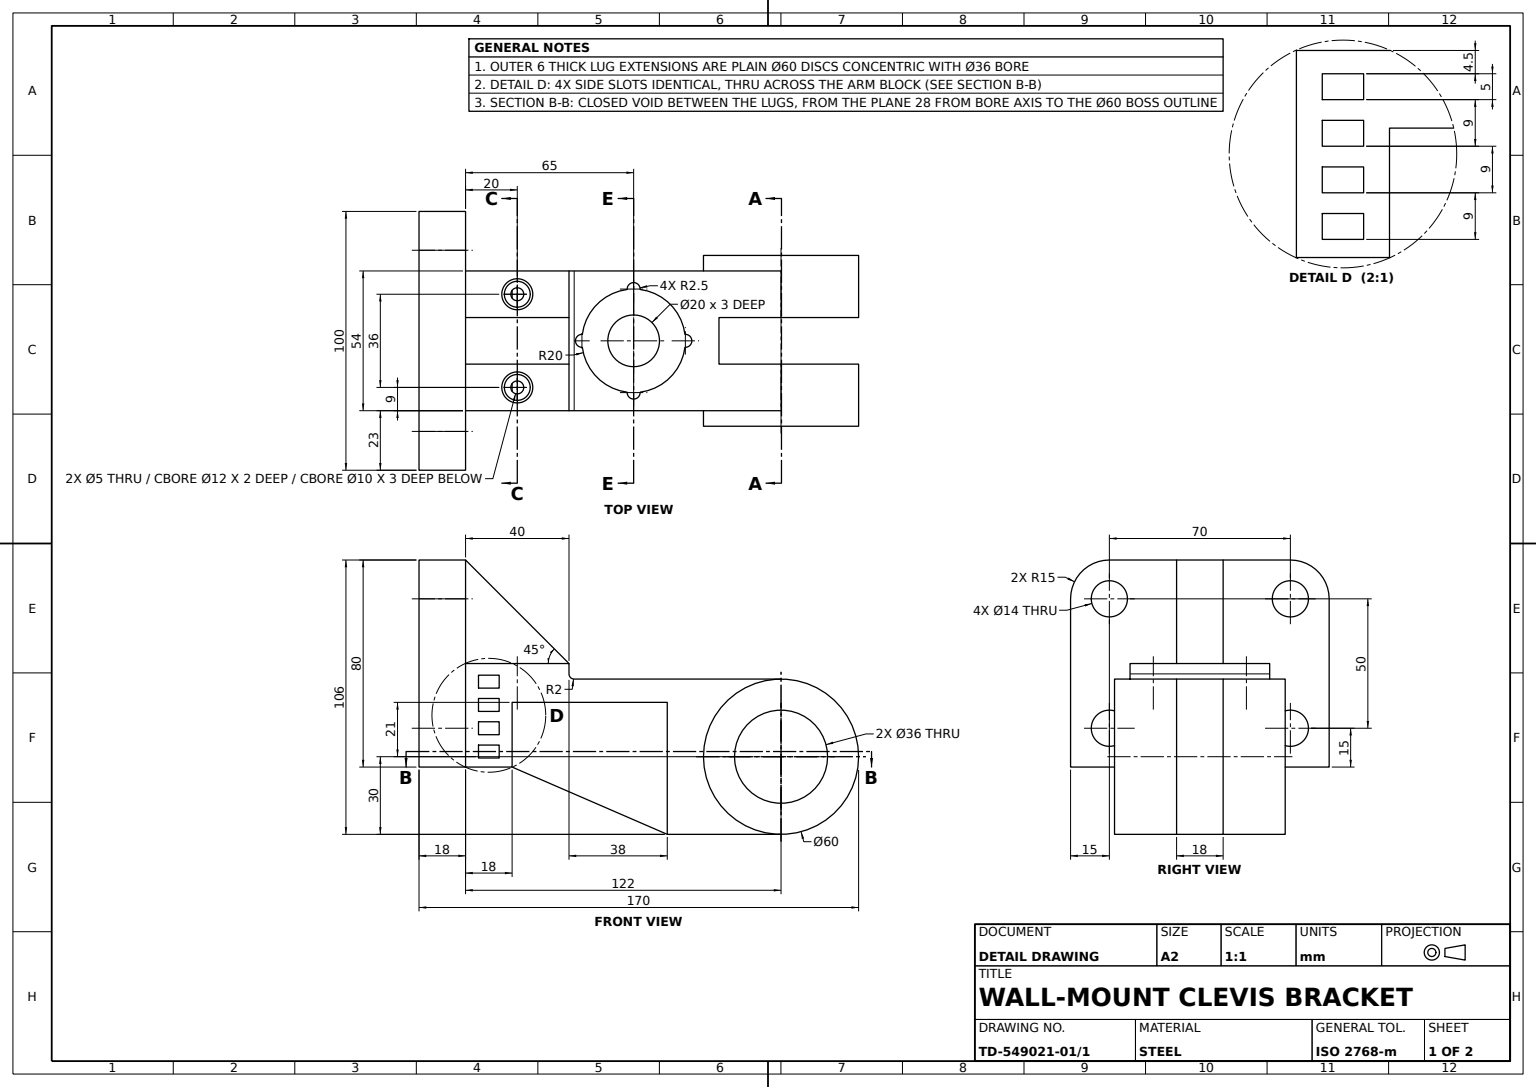
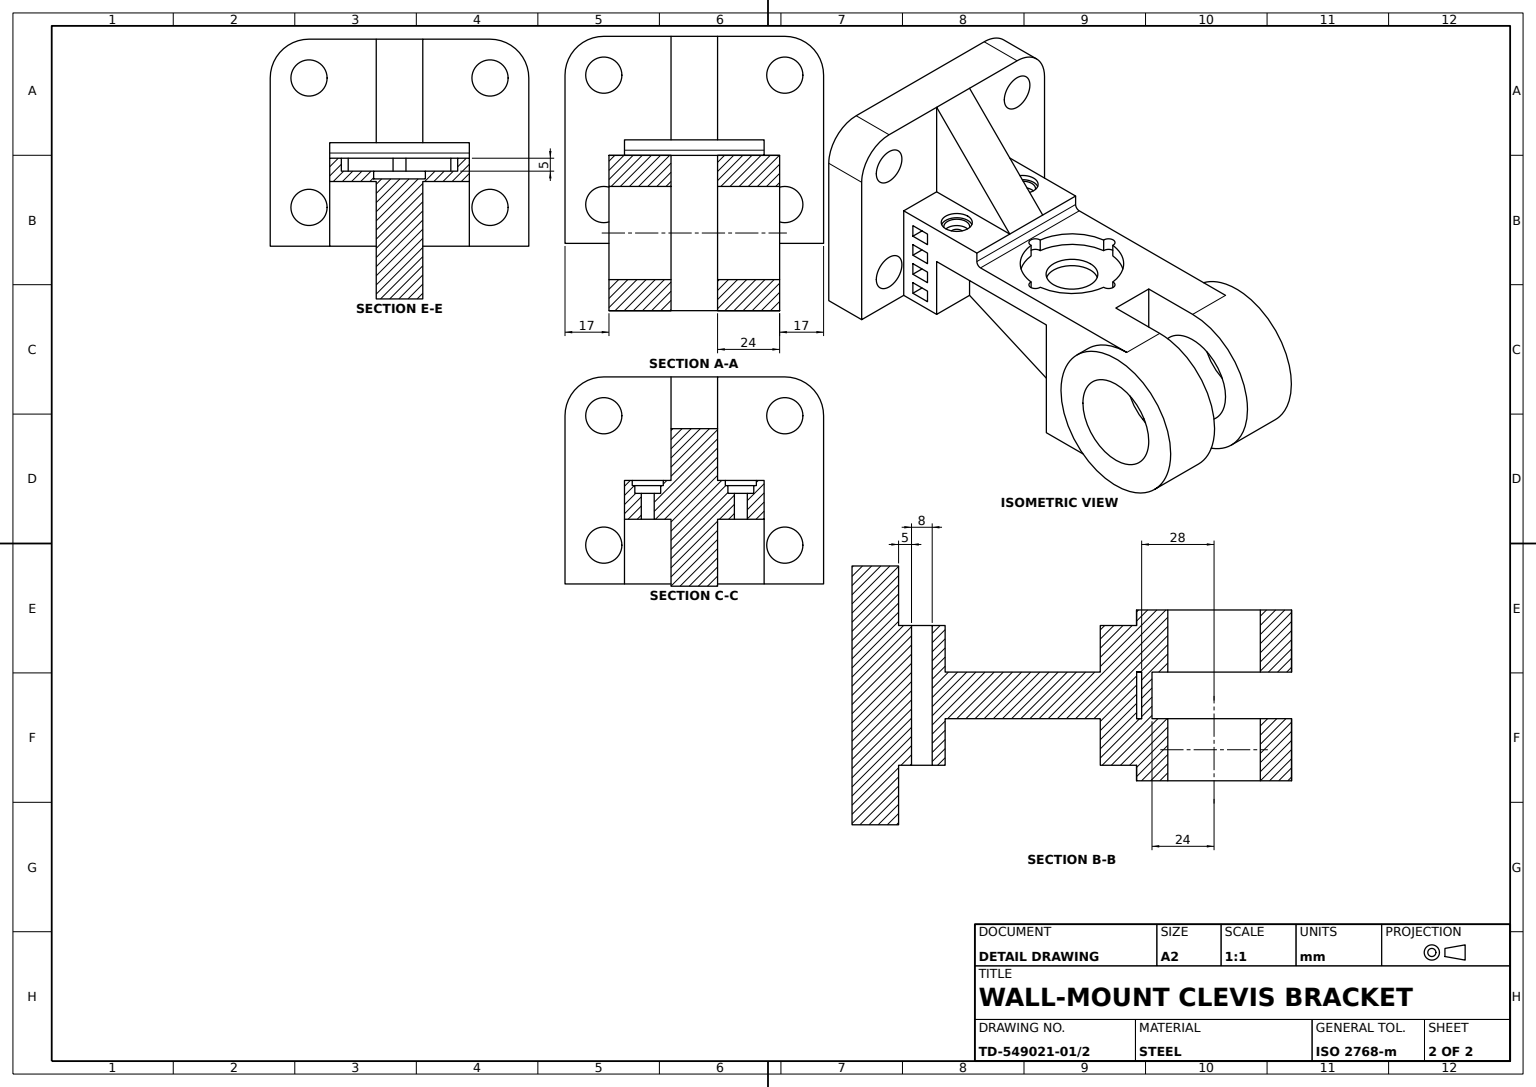
solid
v1 (38,-2,-12)
v2 (38,-2,-24)
e1 v1 v2 CIRCLE(AX(P(38,-2,-18),D(0,1,0),D(0,0,1)),6)
e2 v2 v1 CIRCLE(AX(P(38,-2,-18),D(0,1,0),D(0,0,1)),6)
v3 (38,-2,-23)
v4 (38,-2,-13)
e3 v3 v4 CIRCLE(AX(P(38,-2,-18),D(0,-1,0),D(0,0,1)),5)
e4 v4 v3 CIRCLE(AX(P(38,-2,-18),D(0,-1,0),D(0,0,1)),5)
face PLANE(AX(P(38,-2,-18),D(0,1,0),D(0,0,1))) [e1 e2] [e3 e4]
v5 (38,-5,-13)
v6 (38,-5,-23)
e5 v5 v6 CIRCLE(AX(P(38,-5,-18),D(0,1,0),D(0,0,1)),5)
e6 v5 v4 LINE
e7 v6 v3 LINE
face CYL(AX(P(38,-5,-18),D(0,1,0),D(0,0,1)),5) rev [-e5 e6 -e3 -e7]
v7 (0,25,-28)
v8 (18,25,-28)
e8 v7 v8 LINE
v9 (18,25,-42)
e9 v8 v9 CIRCLE(AX(P(18,25,-35),D(1,0,0),D(0,0,-1)),7)
v10 (0,25,-42)
e10 v10 v9 LINE
e11 v7 v10 CIRCLE(AX(P(0,25,-35),D(1,0,0),D(0,0,-1)),7)
face CYL(AX(P(0,25,-35),D(1,0,0),D(0,0,-1)),7) rev [e8 e9 -e10 -e11]
v11 (85.495112,-11,-19.84375)
v12 (85.495112,-6,-19.84375)
e12 v11 v12 LINE
v13 (80.504888,-6,-19.84375)
e13 v12 v13 CIRCLE(AX(P(83,-6,-20),D(0,1,0),D(0,0,1)),2.5)
v14 (80.504888,-11,-19.84375)
e14 v14 v13 LINE
e15 v11 v14 CIRCLE(AX(P(83,-11,-20),D(0,1,0),D(0,0,1)),2.5)
face CYL(AX(P(83,-11,-20),D(0,1,0),D(0,0,1)),2.5) rev [e12 e13 -e14 -e15]
v15 (96,-15,9)
v16 (96,-15,27)
e16 v15 v16 LINE
v17 (96,-66,9)
e17 v17 v15 LINE
v18 (96,-66,27)
e18 v17 v18 LINE
e19 v16 v18 LINE
face PLANE(AX(P(96,0,-27),D(-1,0,0),D(0,0,1))) [-e16 -e17 e18 -e19]
v19 (38,-15,-20.5)
v20 (38,-5,-20.5)
e20 v19 v20 LINE
v21 (38,-15,-15.5)
e21 v21 v19 CIRCLE(AX(P(38,-15,-18),D(0,1,0),D(0,0,1)),2.5)
v22 (38,-5,-15.5)
e22 v21 v22 LINE
e23 v20 v22 CIRCLE(AX(P(38,-5,-18),D(0,-1,0),D(0,0,1)),2.5)
face CYL(AX(P(38,-15,-18),D(0,1,0),D(0,0,1)),2.5) rev [-e20 -e21 e22 -e23]
v23 (85.495112,-6,19.84375)
v24 (102.84375,-6,2.495112)
e24 v23 v24 CIRCLE(AX(P(83,-6,0),D(0,1,0),D(0,0,1)),20)
v25 (102.84375,-11,2.495112)
e25 v25 v24 LINE
v26 (85.495112,-11,19.84375)
e26 v26 v25 CIRCLE(AX(P(83,-11,0),D(0,1,0),D(0,0,1)),20)
e27 v26 v23 LINE
face CYL(AX(P(83,-11,0),D(0,1,0),D(0,0,1)),20) rev [e24 -e25 -e26 e27]
v27 (38,0,-12)
e28 v1 v27 LINE
v28 (38,0,-24)
e29 v27 v28 CIRCLE(AX(P(38,0,-18),D(0,1,0),D(0,0,1)),6)
e30 v2 v28 LINE
face CYL(AX(P(38,-2,-18),D(0,1,0),D(0,0,1)),6) rev [-e1 e28 e29 -e30]
v29 (38,-2,12)
v30 (38,0,12)
e31 v29 v30 LINE
v31 (38,0,24)
e32 v30 v31 CIRCLE(AX(P(38,0,18),D(0,1,0),D(0,0,1)),6)
v32 (38,-2,24)
e33 v32 v31 LINE
e34 v29 v32 CIRCLE(AX(P(38,-2,18),D(0,1,0),D(0,0,1)),6)
face CYL(AX(P(38,-2,18),D(0,1,0),D(0,0,1)),6) rev [e31 e32 -e33 -e34]
v33 (58,0,9)
v34 (58,0,-9)
e35 v33 v34 LINE
v35 (58,0,27)
e36 v35 v33 LINE
v36 (58,-4,27)
e37 v36 v35 LINE
v37 (58,-4,-27)
e38 v36 v37 LINE
v38 (58,0,-27)
e39 v37 v38 LINE
e40 v34 v38 LINE
face PLANE(AX(P(58,-15,-27),D(1,0,0),D(0,0,-1))) [-e35 -e36 -e37 e38 e39 -e40]
v39 (110,-36,27)
v40 (110,-36,33)
e41 v39 v40 LINE
v41 (140,-66,27)
e42 v39 v41 CIRCLE(AX(P(140,-36,27),D(0,0,1),D(1,0,0)),30)
v42 (140,-66,9)
e43 v42 v41 LINE
v43 (170,-36,9)
e44 v42 v43 CIRCLE(AX(P(140,-36,9),D(0,0,1),D(1,0,0)),30)
v44 (170,-36,33)
e45 v43 v44 LINE
e46 v40 v44 CIRCLE(AX(P(140,-36,33),D(0,0,1),D(1,0,0)),30)
face CYL(AX(P(140,-36,9),D(0,0,1),D(1,0,0)),30) [-e41 e42 -e43 e44 e45 -e46]
v45 (60,-6,27)
e47 v45 v36 CIRCLE(AX(P(60,-4,27),D(0,0,-1),D(-1,0,0)),2)
v46 (60,-6,-27)
e48 v46 v45 LINE
e49 v37 v46 CIRCLE(AX(P(60,-4,-27),D(0,0,1),D(-1,0,0)),2)
face CYL(AX(P(60,-4,-27),D(0,0,-1),D(-1,0,0)),2) rev [-e38 -e47 -e48 -e49]
v47 (0,-25,28)
v48 (18,-25,28)
e50 v47 v48 LINE
v49 (0,-25,42)
e51 v49 v47 CIRCLE(AX(P(0,-25,35),D(1,0,0),D(0,0,-1)),7)
v50 (18,-25,42)
e52 v49 v50 LINE
e53 v50 v48 CIRCLE(AX(P(18,-25,35),D(1,0,0),D(0,0,-1)),7)
face CYL(AX(P(0,-25,35),D(1,0,0),D(0,0,-1)),7) rev [-e50 -e51 e52 e53]
v51 (18,-25,-42)
v52 (18,-25,-28)
e54 v51 v52 CIRCLE(AX(P(18,-25,-35),D(1,0,0),D(0,0,-1)),7)
v53 (0,-25,-28)
e55 v53 v52 LINE
v54 (0,-25,-42)
e56 v54 v53 CIRCLE(AX(P(0,-25,-35),D(1,0,0),D(0,0,-1)),7)
e57 v54 v51 LINE
face CYL(AX(P(0,-25,-35),D(1,0,0),D(0,0,-1)),7) rev [e54 -e55 -e56 e57]
e58 v10 v7 CIRCLE(AX(P(0,25,-35),D(1,0,0),D(0,0,-1)),7)
e59 v9 v8 CIRCLE(AX(P(18,25,-35),D(1,0,0),D(0,0,-1)),7)
face CYL(AX(P(0,25,-35),D(1,0,0),D(0,0,-1)),7) rev [-e58 e10 e59 -e8]
e60 v52 v51 CIRCLE(AX(P(18,-25,-35),D(1,0,0),D(0,0,-1)),7)
v55 (18,0,-27)
v56 (18,-40,-27)
e61 v55 v56 LINE
v57 (18,-40,-50)
e62 v56 v57 LINE
v58 (18,25,-50)
e63 v57 v58 LINE
v59 (18,40,-35)
e64 v58 v59 CIRCLE(AX(P(18,25,-35),D(1,0,0),D(0,0,-1)),15)
v60 (18,40,-9)
e65 v59 v60 LINE
v61 (18,0,-9)
e66 v60 v61 LINE
e67 v55 v61 LINE
face PLANE(AX(P(18,25,35),D(1,0,0),D(0,0,-1))) [-e59 -e9] [-e60 -e54] [e61 e62 e63 e64 e65 e66 -e67]
e68 v53 v54 CIRCLE(AX(P(0,-25,-35),D(1,0,0),D(0,0,-1)),7)
v62 (0,-40,-50)
v63 (0,25,-50)
e69 v62 v63 LINE
v64 (0,-40,50)
e70 v64 v62 LINE
v65 (0,25,50)
e71 v65 v64 LINE
v66 (0,40,35)
e72 v66 v65 CIRCLE(AX(P(0,25,35),D(1,0,0),D(0,0,-1)),15)
v67 (0,40,-35)
e73 v67 v66 LINE
e74 v63 v67 CIRCLE(AX(P(0,25,-35),D(1,0,0),D(0,0,-1)),15)
v68 (0,25,42)
v69 (0,25,28)
e75 v68 v69 CIRCLE(AX(P(0,25,35),D(1,0,0),D(0,0,-1)),7)
e76 v69 v68 CIRCLE(AX(P(0,25,35),D(1,0,0),D(0,0,-1)),7)
e77 v47 v49 CIRCLE(AX(P(0,-25,35),D(1,0,0),D(0,0,-1)),7)
face PLANE(AX(P(0,25,35),D(1,0,0),D(0,0,-1))) rev [e56 e68] [-e69 -e70 -e71 -e72 -e73 -e74] [e11 e58] [e75 e76] [e77 e51]
v70 (18,25,50)
e78 v70 v65 LINE
v71 (18,40,35)
e79 v71 v70 CIRCLE(AX(P(18,25,35),D(1,0,0),D(0,0,-1)),15)
e80 v71 v66 LINE
face CYL(AX(P(18,25,35),D(-1,0,0),D(0,0,1)),15) [-e78 -e79 e80 e72]
v72 (116,-6,9)
v73 (140,-6,9)
e81 v72 v73 LINE
e82 v43 v73 CIRCLE(AX(P(140,-36,9),D(0,0,1),D(1,0,0)),30)
v74 (116,-66,9)
e83 v74 v42 LINE
e84 v74 v72 LINE
v75 (122,-36,9)
v76 (158,-36,9)
e85 v75 v76 CIRCLE(AX(P(140,-36,9),D(0,0,1),D(1,0,0)),18)
e86 v76 v75 CIRCLE(AX(P(140,-36,9),D(0,0,1),D(1,0,0)),18)
face PLANE(AX(P(0,0,9),D(0,0,1),D(1,0,0))) rev [e81 -e82 -e44 -e83 e84] [e85 e86]
v77 (18,0,9)
e87 v33 v77 LINE
v78 (18,0,27)
e88 v77 v78 LINE
e89 v78 v35 LINE
e90 v31 v30 CIRCLE(AX(P(38,0,18),D(0,1,0),D(0,0,1)),6)
face PLANE(AX(P(0,0,0),D(0,-1,0),D(0,0,-1))) rev [e36 e87 e88 e89] [-e32 -e90]
e91 v34 v61 LINE
e92 v55 v38 LINE
e93 v28 v27 CIRCLE(AX(P(38,0,-18),D(0,1,0),D(0,0,1)),6)
face PLANE(AX(P(0,0,0),D(0,-1,0),D(0,0,-1))) rev [-e91 e40 -e92 e67] [-e29 -e93]
v79 (31,-27.5,-27)
v80 (31,-27.5,27)
e94 v79 v80 LINE
v81 (23,-27.5,-27)
e95 v79 v81 LINE
v82 (23,-27.5,27)
e96 v81 v82 LINE
e97 v82 v80 LINE
face PLANE(AX(P(23,-27.5,-50),D(0,-1,0),D(0,0,-1))) rev [-e94 e95 e96 e97]
v83 (122,-36,33)
e98 v75 v83 LINE
v84 (158,-36,33)
e99 v76 v84 LINE
e100 v84 v83 CIRCLE(AX(P(140,-36,33),D(0,0,1),D(1,0,0)),18)
face CYL(AX(P(140,-36,9),D(0,0,1),D(1,0,0)),18) rev [-e98 -e86 e99 e100]
v85 (140,-66,-27)
v86 (140,-66,-9)
e101 v85 v86 LINE
v87 (110,-36,-27)
e102 v85 v87 CIRCLE(AX(P(140,-36,-27),D(0,0,-1),D(-1,0,0)),30)
v88 (110,-36,-33)
e103 v87 v88 LINE
v89 (170,-36,-33)
e104 v89 v88 CIRCLE(AX(P(140,-36,-33),D(0,0,-1),D(-1,0,0)),30)
v90 (170,-36,-9)
e105 v90 v89 LINE
e106 v90 v86 CIRCLE(AX(P(140,-36,-9),D(0,0,-1),D(-1,0,0)),30)
face CYL(AX(P(140,-36,-9),D(0,0,-1),D(-1,0,0)),30) [-e101 e102 e103 -e104 -e105 e106]
v91 (36,-40,-9)
v92 (36,-40,-27)
e107 v91 v92 LINE
v93 (36,-40,9)
e108 v91 v93 LINE
v94 (36,-40,27)
e109 v94 v93 LINE
v95 (18,-40,27)
e110 v95 v94 LINE
v96 (18,-40,50)
e111 v96 v95 LINE
e112 v96 v64 LINE
e113 v57 v62 LINE
e114 v56 v92 LINE
face PLANE(AX(P(18,-40,50),D(0,1,0),D(0,0,1))) rev [-e107 e108 -e109 -e110 -e111 e112 e70 -e113 -e62 e114]
v97 (23,-36.5,-27)
v98 (23,-31.5,-27)
e115 v97 v98 LINE
v99 (23,-31.5,27)
e116 v98 v99 LINE
v100 (23,-36.5,27)
e117 v99 v100 LINE
e118 v97 v100 LINE
face PLANE(AX(P(23,-31.5,-50),D(-1,0,0),D(0,0,1))) rev [e115 e116 e117 -e118]
v101 (96,-66,-27)
e119 v101 v85 LINE
v102 (116,-66,-9)
e120 v86 v102 LINE
e121 v102 v74 LINE
e122 v18 v41 LINE
v103 (96,-66,-9)
e123 v103 v17 LINE
e124 v101 v103 LINE
face PLANE(AX(P(0,-66,-27),D(0,-1,0),D(0,0,-1))) [e119 e101 e120 e121 e83 e43 -e122 -e18 -e123 -e124]
v104 (63.15625,-6,2.495112)
v105 (80.504888,-6,19.84375)
e125 v104 v105 CIRCLE(AX(P(83,-6,0),D(0,1,0),D(0,0,1)),20)
v106 (80.504888,-11,19.84375)
e126 v106 v105 LINE
v107 (63.15625,-11,2.495112)
e127 v107 v106 CIRCLE(AX(P(83,-11,0),D(0,1,0),D(0,0,1)),20)
e128 v107 v104 LINE
face CYL(AX(P(83,-11,0),D(0,1,0),D(0,0,1)),20) rev [e125 -e126 -e127 e128]
face CYL(AX(P(38,-2,-18),D(0,1,0),D(0,0,1)),6) rev [e30 e93 -e28 -e2]
v108 (36,-15,16.5)
v109 (36,-15,9)
e129 v108 v109 LINE
e130 v109 v15 LINE
v110 (36,-15,27)
e131 v110 v16 LINE
v111 (36,-15,19.5)
e132 v110 v111 LINE
v112 (38,-15,20.5)
e133 v111 v112 CIRCLE(AX(P(38,-15,18),D(0,1,0),D(0,0,1)),2.5)
v113 (38,-15,15.5)
e134 v112 v113 CIRCLE(AX(P(38,-15,18),D(0,1,0),D(0,0,1)),2.5)
e135 v113 v108 CIRCLE(AX(P(38,-15,18),D(0,1,0),D(0,0,1)),2.5)
face PLANE(AX(P(0,-15,0),D(0,1,0),D(0,0,1))) rev [e129 e130 e16 -e131 e132 e133 e134 e135]
e136 v93 v109 LINE
e137 v93 v17 LINE
face PLANE(AX(P(85,-13,9),D(0,0,1),D(1,0,0))) [-e130 -e136 e137 e17]
v114 (31,-4.5,27)
v115 (23,-4.5,27)
e138 v114 v115 LINE
v116 (31,-9.5,27)
e139 v116 v114 LINE
v117 (23,-9.5,27)
e140 v117 v116 LINE
e141 v115 v117 LINE
v118 (140,-6,27)
e142 v118 v39 CIRCLE(AX(P(140,-36,27),D(0,0,1),D(1,0,0)),30)
e143 v118 v45 LINE
e144 v78 v95 LINE
e145 v110 v94 LINE
v119 (23,-13.5,27)
v120 (23,-18.5,27)
e146 v119 v120 LINE
v121 (31,-13.5,27)
e147 v121 v119 LINE
v122 (31,-18.5,27)
e148 v122 v121 LINE
e149 v120 v122 LINE
v123 (23,-22.5,27)
e150 v123 v82 LINE
v124 (31,-22.5,27)
e151 v124 v123 LINE
e152 v80 v124 LINE
v125 (31,-31.5,27)
e153 v125 v99 LINE
v126 (31,-36.5,27)
e154 v126 v125 LINE
e155 v100 v126 LINE
face PLANE(AX(P(0,0,27),D(0,0,-1),D(-1,0,0))) rev [-e138 -e139 -e140 -e141] [e19 e122 -e42 -e142 e143 e47 e37 -e89 e144 e110 -e145 e131] [-e146 -e147 -e148 -e149] [-e150 -e151 -e152 -e97] [-e117 -e153 -e154 -e155]
e156 v59 v67 LINE
e157 v58 v63 LINE
face CYL(AX(P(18,25,-35),D(-1,0,0),D(0,0,1)),15) [e74 -e156 -e64 e157]
v127 (96,-15,-9)
e158 v103 v127 LINE
v128 (96,-15,-27)
e159 v128 v127 LINE
e160 v128 v101 LINE
face PLANE(AX(P(96,0,-27),D(-1,0,0),D(0,0,1))) [e158 -e159 e160 e124]
v129 (18,40,9)
e161 v129 v71 LINE
e162 v60 v129 LINE
face PLANE(AX(P(18,40,35),D(0,-1,0),D(0,0,-1))) rev [-e161 -e162 -e65 e156 e73 -e80]
v130 (158,-36,-33)
v131 (122,-36,-33)
e163 v130 v131 CIRCLE(AX(P(140,-36,-33),D(0,0,-1),D(-1,0,0)),18)
e164 v131 v130 CIRCLE(AX(P(140,-36,-33),D(0,0,-1),D(-1,0,0)),18)
e165 v88 v89 CIRCLE(AX(P(140,-36,-33),D(0,0,-1),D(-1,0,0)),30)
face PLANE(AX(P(140,-36,-33),D(0,0,-1),D(-1,0,0))) [-e163 -e164] [e104 e165]
v132 (23,-13.5,-27)
e166 v132 v119 LINE
v133 (23,-18.5,-27)
e167 v133 v120 LINE
e168 v133 v132 LINE
face PLANE(AX(P(23,-13.5,-50),D(-1,0,0),D(0,0,1))) rev [e166 e146 -e167 e168]
v134 (103,-6,-2.5)
v135 (102.84375,-6,-2.495112)
e169 v134 v135 CIRCLE(AX(P(103,-6,0),D(0,1,0),D(0,0,1)),2.5)
v136 (102.84375,-11,-2.495112)
e170 v136 v135 LINE
v137 (103,-11,-2.5)
e171 v137 v136 CIRCLE(AX(P(103,-11,0),D(0,1,0),D(0,0,1)),2.5)
e172 v137 v134 LINE
face CYL(AX(P(103,-11,0),D(0,1,0),D(0,0,1)),2.5) rev [e169 -e170 -e171 e172]
v138 (36,-15,-19.5)
e173 v19 v138 CIRCLE(AX(P(38,-15,-18),D(0,1,0),D(0,0,1)),2.5)
v139 (36,-15,-27)
e174 v138 v139 LINE
e175 v128 v139 LINE
v140 (36,-15,-9)
e176 v140 v127 LINE
v141 (36,-15,-16.5)
e177 v140 v141 LINE
e178 v141 v21 CIRCLE(AX(P(38,-15,-18),D(0,1,0),D(0,0,1)),2.5)
face PLANE(AX(P(0,-15,0),D(0,1,0),D(0,0,1))) rev [e21 e173 e174 -e175 e159 -e176 e177 e178]
v142 (83,-6,22.5)
e179 v105 v142 CIRCLE(AX(P(83,-6,20),D(0,1,0),D(0,0,1)),2.5)
v143 (83,-11,22.5)
e180 v143 v142 LINE
e181 v106 v143 CIRCLE(AX(P(83,-11,20),D(0,1,0),D(0,0,1)),2.5)
face CYL(AX(P(83,-11,20),D(0,1,0),D(0,0,1)),2.5) rev [e179 -e180 -e181 e126]
e182 v60 v34 LINE
face PLANE(AX(P(29,0,-9),D(0,0,1),D(1,0,0))) rev [e182 e91 -e66]
e183 v135 v12 CIRCLE(AX(P(83,-6,0),D(0,1,0),D(0,0,1)),20)
e184 v136 v11 CIRCLE(AX(P(83,-11,0),D(0,1,0),D(0,0,1)),20)
face CYL(AX(P(83,-11,0),D(0,1,0),D(0,0,1)),20) rev [e183 -e12 -e184 e170]
v144 (63.15625,-6,-2.495112)
e185 v13 v144 CIRCLE(AX(P(83,-6,0),D(0,1,0),D(0,0,1)),20)
v145 (63.15625,-11,-2.495112)
e186 v145 v144 LINE
e187 v14 v145 CIRCLE(AX(P(83,-11,0),D(0,1,0),D(0,0,1)),20)
face CYL(AX(P(83,-11,0),D(0,1,0),D(0,0,1)),20) rev [e185 -e186 -e187 e14]
e188 v141 v138 LINE
e189 v138 v141 CIRCLE(AX(P(38,-15,-18),D(0,1,0),D(0,0,1)),2.5)
face PLANE(AX(P(38,-15,-18),D(0,1,0),D(0,0,1))) [e188 e189]
e190 v129 v33 LINE
face PLANE(AX(P(18,40,0),D(-0.707106781,-0.707106781,0),D(0.707106781,-0.707106781,0))) rev [-e182 e162 e190 e35]
v146 (140,-6,-9)
e191 v146 v90 CIRCLE(AX(P(140,-36,-9),D(0,0,-1),D(-1,0,0)),30)
v147 (116,-6,-9)
e192 v146 v147 LINE
e193 v102 v147 LINE
v148 (158,-36,-9)
v149 (122,-36,-9)
e194 v148 v149 CIRCLE(AX(P(140,-36,-9),D(0,0,-1),D(-1,0,0)),18)
e195 v149 v148 CIRCLE(AX(P(140,-36,-9),D(0,0,-1),D(-1,0,0)),18)
face PLANE(AX(P(140,-36,-9),D(0,0,-1),D(-1,0,0))) rev [-e106 -e191 e192 -e193 -e120] [e194 e195]
e196 v48 v50 CIRCLE(AX(P(18,-25,35),D(1,0,0),D(0,0,-1)),7)
face CYL(AX(P(0,-25,35),D(1,0,0),D(0,0,-1)),7) rev [-e77 e50 e196 -e52]
v150 (38,-5,15.5)
e197 v113 v150 LINE
v151 (38,-5,20.5)
e198 v112 v151 LINE
e199 v150 v151 CIRCLE(AX(P(38,-5,18),D(0,-1,0),D(0,0,1)),2.5)
face CYL(AX(P(38,-15,18),D(0,1,0),D(0,0,1)),2.5) rev [-e197 -e134 e198 -e199]
v152 (23,-9.5,-27)
v153 (23,-4.5,-27)
e200 v152 v153 LINE
e201 v153 v115 LINE
e202 v152 v117 LINE
face PLANE(AX(P(23,-4.5,-50),D(-1,0,0),D(0,0,1))) rev [e200 e201 e141 -e202]
v154 (83,-11,10)
v155 (83,-11,-10)
e203 v154 v155 CIRCLE(AX(P(83,-11,0),D(0,1,0),D(0,0,1)),10)
v156 (83,-14,-10)
e204 v156 v155 LINE
v157 (83,-14,10)
e205 v157 v156 CIRCLE(AX(P(83,-14,0),D(0,1,0),D(0,0,1)),10)
e206 v157 v154 LINE
face CYL(AX(P(83,-14,0),D(0,1,0),D(0,0,1)),10) rev [e203 -e204 -e205 e206]
v158 (31,-36.5,-27)
e207 v158 v126 LINE
e208 v158 v97 LINE
face PLANE(AX(P(23,-36.5,-50),D(0,-1,0),D(1,0,0))) rev [e118 e155 -e207 e208]
v159 (31,-4.5,-27)
v160 (31,-9.5,-27)
e209 v159 v160 LINE
e210 v160 v116 LINE
e211 v159 v114 LINE
face PLANE(AX(P(31,-4.5,-50),D(1,0,0),D(0,0,-1))) rev [e209 e210 e139 -e211]
v161 (103,-6,2.5)
e212 v24 v161 CIRCLE(AX(P(103,-6,0),D(0,1,0),D(0,0,1)),2.5)
v162 (103,-11,2.5)
e213 v162 v161 LINE
e214 v25 v162 CIRCLE(AX(P(103,-11,0),D(0,1,0),D(0,0,1)),2.5)
face CYL(AX(P(103,-11,0),D(0,1,0),D(0,0,1)),2.5) rev [e25 e212 -e213 -e214]
e215 v70 v96 LINE
face PLANE(AX(P(18,-40,50),D(0,0,-1),D(-1,0,0))) rev [e71 -e112 -e215 e78]
e216 v108 v111 CIRCLE(AX(P(38,-15,18),D(0,1,0),D(0,0,1)),2.5)
e217 v111 v108 LINE
face PLANE(AX(P(38,-15,18),D(0,1,0),D(0,0,1))) [e216 e217]
v163 (63,-6,2.5)
e218 v163 v104 CIRCLE(AX(P(63,-6,0),D(0,1,0),D(0,0,1)),2.5)
v164 (63,-6,-2.5)
e219 v164 v163 CIRCLE(AX(P(63,-6,0),D(0,1,0),D(0,0,1)),2.5)
e220 v144 v164 CIRCLE(AX(P(63,-6,0),D(0,1,0),D(0,0,1)),2.5)
e221 v161 v134 CIRCLE(AX(P(103,-6,0),D(0,1,0),D(0,0,1)),2.5)
e222 v142 v23 CIRCLE(AX(P(83,-6,20),D(0,1,0),D(0,0,1)),2.5)
e223 v73 v118 LINE
e224 v147 v72 LINE
v165 (140,-6,-27)
e225 v165 v146 LINE
e226 v165 v46 LINE
face PLANE(AX(P(0,-6,-27),D(0,1,0),D(0,0,1))) [-e179 -e125 -e218 -e219 -e220 -e185 -e13 -e183 -e169 -e221 -e212 -e24 -e222] [-e143 -e223 -e81 -e224 -e192 -e225 e226 e48]
v166 (38,-2,23)
v167 (38,-2,13)
e227 v166 v167 CIRCLE(AX(P(38,-2,18),D(0,-1,0),D(0,0,1)),5)
e228 v167 v166 CIRCLE(AX(P(38,-2,18),D(0,-1,0),D(0,0,1)),5)
e229 v32 v29 CIRCLE(AX(P(38,-2,18),D(0,1,0),D(0,0,1)),6)
face PLANE(AX(P(38,-2,18),D(0,1,0),D(0,0,1))) [e227 e228] [e34 e229]
v168 (31,-18.5,-27)
e230 v168 v122 LINE
e231 v168 v133 LINE
face PLANE(AX(P(23,-18.5,-50),D(0,-1,0),D(1,0,0))) rev [-e230 e231 e167 e149]
v169 (63,-11,2.5)
e232 v169 v107 CIRCLE(AX(P(63,-11,0),D(0,1,0),D(0,0,1)),2.5)
e233 v169 v163 LINE
face CYL(AX(P(63,-11,0),D(0,1,0),D(0,0,1)),2.5) rev [-e128 -e232 e233 e218]
e234 v83 v84 CIRCLE(AX(P(140,-36,33),D(0,0,1),D(1,0,0)),18)
face CYL(AX(P(140,-36,9),D(0,0,1),D(1,0,0)),18) rev [-e99 -e85 e98 e234]
face PLANE(AX(P(36,0,0),D(-1,0,0),D(0,0,1))) rev [-e132 e145 e109 e136 -e129 -e217]
e235 v91 v140 LINE
e236 v91 v103 LINE
face PLANE(AX(P(85,-13,-9),D(0,0,1),D(1,0,0))) rev [e235 e176 -e158 -e236]
face PLANE(AX(P(18,-40,-50),D(0,0,1),D(1,0,0))) rev [e69 -e157 -e63 e113]
e237 v148 v130 LINE
e238 v149 v131 LINE
face CYL(AX(P(140,-36,-9),D(0,0,-1),D(-1,0,0)),18) rev [-e237 -e195 e238 e164]
face CYL(AX(P(38,-2,18),D(0,1,0),D(0,0,1)),6) rev [e33 e90 -e31 -e229]
v170 (38,-5,23)
e239 v170 v166 LINE
v171 (38,-5,13)
e240 v171 v167 LINE
e241 v170 v171 CIRCLE(AX(P(38,-5,18),D(0,1,0),D(0,0,1)),5)
face CYL(AX(P(38,-5,18),D(0,1,0),D(0,0,1)),5) rev [e239 -e228 -e240 -e241]
v172 (31,-13.5,-27)
e242 v132 v172 LINE
e243 v172 v121 LINE
face PLANE(AX(P(23,-13.5,-50),D(0,1,0),D(0,0,1))) rev [e147 -e166 e242 e243]
v173 (18,25,28)
e244 v69 v173 LINE
v174 (18,25,42)
e245 v173 v174 CIRCLE(AX(P(18,25,35),D(1,0,0),D(0,0,-1)),7)
e246 v68 v174 LINE
face CYL(AX(P(0,25,35),D(1,0,0),D(0,0,-1)),7) rev [-e76 e244 e245 -e246]
e247 v162 v137 CIRCLE(AX(P(103,-11,0),D(0,1,0),D(0,0,1)),2.5)
face CYL(AX(P(103,-11,0),D(0,1,0),D(0,0,1)),2.5) rev [e213 e221 -e172 -e247]
e248 v6 v5 CIRCLE(AX(P(38,-5,-18),D(0,1,0),D(0,0,1)),5)
face CYL(AX(P(38,-5,-18),D(0,1,0),D(0,0,1)),5) rev [-e4 -e6 -e248 e7]
e249 v44 v40 CIRCLE(AX(P(140,-36,33),D(0,0,1),D(1,0,0)),30)
face CYL(AX(P(140,-36,9),D(0,0,1),D(1,0,0)),30) [e41 -e249 -e45 e82 e223 e142]
face CYL(AX(P(0,-25,-35),D(1,0,0),D(0,0,-1)),7) rev [e55 e60 -e57 -e68]
e250 v174 v173 CIRCLE(AX(P(18,25,35),D(1,0,0),D(0,0,-1)),7)
face CYL(AX(P(0,25,35),D(1,0,0),D(0,0,-1)),7) rev [-e75 e246 e250 -e244]
v175 (63,-11,-2.5)
e251 v145 v175 CIRCLE(AX(P(63,-11,0),D(0,1,0),D(0,0,1)),2.5)
e252 v175 v164 LINE
face CYL(AX(P(63,-11,0),D(0,1,0),D(0,0,1)),2.5) rev [-e251 e186 e220 -e252]
v176 (31,-31.5,-27)
e253 v176 v158 LINE
e254 v98 v176 LINE
e255 v172 v168 LINE
v177 (31,-22.5,-27)
e256 v177 v79 LINE
v178 (23,-22.5,-27)
e257 v178 v177 LINE
e258 v81 v178 LINE
e259 v153 v159 LINE
e260 v160 v152 LINE
e261 v139 v92 LINE
e262 v87 v165 CIRCLE(AX(P(140,-36,-27),D(0,0,-1),D(-1,0,0)),30)
face PLANE(AX(P(0,0,-27),D(0,0,-1),D(-1,0,0))) [-e253 -e254 -e115 -e208] [-e255 -e242 -e168 -e231] [-e95 -e256 -e257 -e258] [-e209 -e259 -e200 -e260] [e175 e261 -e114 -e61 e92 -e39 e49 -e226 -e262 -e102 -e119 -e160]
e263 v171 v170 CIRCLE(AX(P(38,-5,18),D(0,1,0),D(0,0,1)),5)
face CYL(AX(P(38,-5,18),D(0,1,0),D(0,0,1)),5) rev [-e239 -e263 e240 -e227]
face PLANE(AX(P(116,-66,-9),D(-1,0,0),D(0,0,1))) rev [-e121 e193 e224 -e84]
e264 v156 v157 CIRCLE(AX(P(83,-14,0),D(0,1,0),D(0,0,1)),10)
face PLANE(AX(P(83,-14,0),D(0,1,0),D(0,0,1))) [e264 e205]
e265 v143 v26 CIRCLE(AX(P(83,-11,20),D(0,1,0),D(0,0,1)),2.5)
face CYL(AX(P(83,-11,20),D(0,1,0),D(0,0,1)),2.5) rev [e222 -e27 -e265 e180]
e266 v22 v20 CIRCLE(AX(P(38,-5,-18),D(0,-1,0),D(0,0,1)),2.5)
face PLANE(AX(P(38,-5,-18),D(0,1,0),D(0,0,1))) [e23 e266] [e5 e248]
face CYL(AX(P(140,-36,-9),D(0,0,-1),D(-1,0,0)),30) [-e103 e262 e225 e191 e105 -e165]
face PLANE(AX(P(0,0,33),D(0,0,1),D(1,0,0))) [e46 e249] [-e234 -e100]
e267 v151 v150 CIRCLE(AX(P(38,-5,18),D(0,-1,0),D(0,0,1)),2.5)
face PLANE(AX(P(38,-5,18),D(0,1,0),D(0,0,1))) [e241 e263] [e267 e199]
e268 v178 v123 LINE
face PLANE(AX(P(23,-22.5,-50),D(-1,0,0),D(0,0,1))) rev [e150 -e96 e258 e268]
face PLANE(AX(P(23,-9.5,-50),D(0,-1,0),D(1,0,0))) rev [-e210 e260 e202 e140]
e269 v155 v154 CIRCLE(AX(P(83,-11,0),D(0,1,0),D(0,0,1)),10)
e270 v175 v169 CIRCLE(AX(P(63,-11,0),D(0,1,0),D(0,0,1)),2.5)
face PLANE(AX(P(83,-11,-10),D(0,1,0),D(0,0,1))) [-e203 -e269] [e187 e251 e270 e232 e127 e181 e265 e26 e214 e247 e171 e184 e15]
e271 v129 v77 LINE
face PLANE(AX(P(18,25,35),D(1,0,0),D(0,0,-1))) [e215 e111 -e144 -e88 -e271 e161 e79] [-e245 -e250] [-e196 -e53]
face CYL(AX(P(38,-15,18),D(0,1,0),D(0,0,1)),2.5) rev [-e267 -e198 -e133 -e216 -e135 e197]
face CYL(AX(P(83,-14,0),D(0,1,0),D(0,0,1)),10) rev [-e264 e204 e269 -e206]
e272 v177 v124 LINE
face PLANE(AX(P(23,-22.5,-50),D(0,1,0),D(-1,0,0))) rev [e257 e272 e151 -e268]
face PLANE(AX(P(31,-22.5,-50),D(1,0,0),D(0,0,-1))) rev [e152 -e272 e256 e94]
face PLANE(AX(P(36,0,0),D(-1,0,0),D(0,0,1))) rev [-e177 -e235 e107 -e261 -e174 -e188]
e273 v176 v125 LINE
face PLANE(AX(P(23,-31.5,-50),D(0,1,0),D(0,0,1))) rev [e273 e153 -e116 e254]
face PLANE(AX(P(36,-40,0),D(-0.397607438,-0.917555625,0),D(0.917555625,-0.397607438,0))) [-e108 e236 e123 -e137]
face PLANE(AX(P(23,-4.5,-50),D(0,1,0),D(-1,0,0))) rev [e259 e211 e138 -e201]
face PLANE(AX(P(31,-31.5,-50),D(1,0,0),D(0,0,-1))) rev [e253 e207 e154 -e273]
face PLANE(AX(P(31,-13.5,-50),D(1,0,0),D(0,0,-1))) rev [e148 -e243 e255 e230]
face CYL(AX(P(38,-15,-18),D(0,1,0),D(0,0,1)),2.5) rev [-e173 e20 -e266 -e22 -e178 -e189]
face PLANE(AX(P(29,0,9),D(0,0,1),D(1,0,0))) [-e190 e271 -e87]
face CYL(AX(P(140,-36,-9),D(0,0,-1),D(-1,0,0)),18) rev [e237 e163 -e238 -e194]
face CYL(AX(P(63,-11,0),D(0,1,0),D(0,0,1)),2.5) rev [-e270 e252 e219 -e233]
void
v179 (112,-25.22967,-9)
v180 (112,-25.22967,9)
e274 v179 v180 LINE
v181 (112,-46.77033,-9)
e275 v181 v179 LINE
v182 (112,-46.77033,9)
e276 v182 v181 LINE
e277 v182 v180 LINE
face PLANE(AX(P(112,-84.439089,-9),D(-1,0,0),D(0,0,1))) [-e274 -e275 -e276 e277]
e278 v181 v179 CIRCLE(AX(P(140,-36,-9),D(0,0,-1),D(-1,0,0)),30)
face PLANE(AX(P(140,-36,-9),D(0,0,-1),D(-1,0,0))) rev [-e278 e275]
e279 v180 v182 CIRCLE(AX(P(140,-36,9),D(0,0,1),D(1,0,0)),30)
face CYL(AX(P(140,-36,-27),D(0,0,1),D(1,0,0)),30) rev [e278 e274 e279 e276]
face PLANE(AX(P(0,0,9),D(0,0,1),D(1,0,0))) rev [-e279 -e277]
